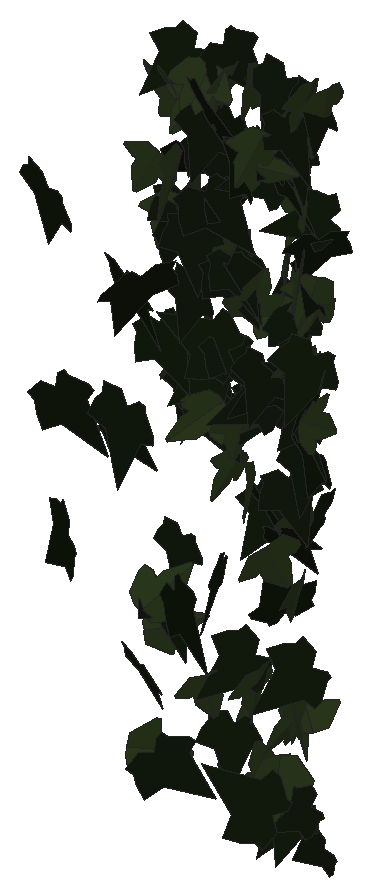
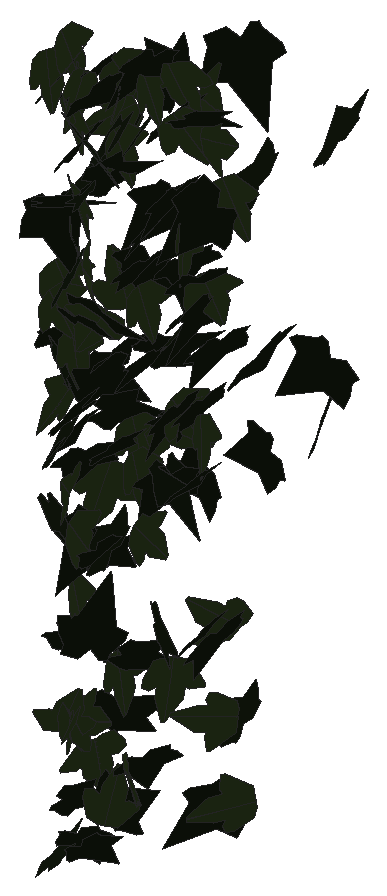
# SketchUp Ruby script. Lengths in inches.
U = 1.inch
M = Sketchup.active_model
def pt(a) = Geom::Point3d.new(a.map { |v| v * U })
def face(e, loops, mat)
  f = e.add_face(loops[0].map { |a| pt(a) })
  loops[1..].each { |l| e.add_face(l.map { |a| pt(a) }).erase! }
  f.material = f.back_material = mat if mat
  f
end
# faces: each face lists its corners as indices into pts; further lists are holes
def faces(e, pts, list, mat = nil) = list.each { |f| face(e, (f[0].is_a?(Array) ? f : [f]).map { |l| l.map { |i| pts[i] } }, mat) }
# xy, xz, yz: faces in a plane at the given z, y or x. An outline is a flat list of corners, or four numbers for a rectangle; further outlines are holes
def ring(l) = l.size == 4 ? [[l[0], l[1]], [l[2], l[1]], [l[2], l[3]], [l[0], l[3]]] : l.each_slice(2).to_a
def flat(e, list, mat, &to3) = list.each { |f| face(e, (f[0].is_a?(Array) ? f : [f]).map { |l| ring(l).map { |u, v| to3.(u, v) } }, mat) }
def xy(e, z, list, mat = nil) = flat(e, list, mat) { |x, y| [x, y, z] }
def xz(e, y, list, mat = nil) = flat(e, list, mat) { |x, z| [x, y, z] }
def yz(e, x, list, mat = nil) = flat(e, list, mat) { |y, z| [x, y, z] }
def lines(e, pts, list) = list.each { |a, b| e.add_line(pt(pts[a]), pt(pts[b])) }
# prism: a flat outline (further loops are holes) pulled along v
def prism(e, loops, v, mat = nil)
  f = face(e, loops, mat); d = Geom::Vector3d.new(v.map { |x| x * U })
  f.pushpull(f.normal.samedirection?(d) ? d.length : -d.length)
end
def box(e, o, s, mat = nil) = prism(e, [[o, [o[0] + s[0], o[1], o[2]], [o[0] + s[0], o[1] + s[1], o[2]], [o[0], o[1] + s[1], o[2]]]], [0, 0, s[2]], mat)
def at(x, y, z, deg = 0) = Geom::Transformation.translation(pt([x, y, z])) * Geom::Transformation.rotation(ORIGIN, Z_AXIS, deg.degrees)
def axes(o, x, y, z) = Geom::Transformation.new([*x, 0, *y, 0, *z, 0, *pt(o).to_a, 1])
def part(name) = M.definitions.add(name)
# library, detail: a bought-in or finely detailed component or shape, given as its bounding box
def library(name, o, s) = part(name).tap { |d| box(d.entities, o, s) }
def detail(e, o, s) = box(e.add_group.entities, o, s)
def put(e, d, t, mat = nil) = e.add_instance(d, t).tap { |i| i.material = mat if mat }
def group(e, t, mat = nil) = e.add_group.tap { |g| g.transformation = t; g.material = mat if mat }.entities
root = M.entities
M.materials.add("efeu1").color = [18, 25, 13]
M.materials.add("efeu2").color = [43, 57, 29]
c1 = part("ivyleaf_9")
p = [[1.54,2.16,1.25],[1.36,2.04,1.19],[-0.21,0.99,0.68],[-0.71,1.11,0.82],[-0.85,0.86,0.67],[-0.8,0.17,0.21],
  [-0.9,-0.01,0.1],[-0.67,-0.16,-0.02],[-0.08,-0.08,-0.05],[-0.03,-0.6,-0.4],[0.65,-0.88,-0.66],[0.83,-0.6,-0.49],
  [1.29,-0.42,-0.43],[1.8125,-0.07,-0.26],[1.21,0.44,0.15]]
faces(c1.entities,p,[[0,1,2,3,4,5,6,7,8,9,10,11,12,13,14]],"efeu1")
c2 = part("ivyleaf_10")
p = [[0,0.5,-0.03],[-0.0625,2.02,-0.43],[-0.19,2.01,-0.46],[-0.54,1.05,-0.29],[-0.52,0.625,-0.18],[-0.83,0.76,-0.28],
  [-1.16,0.64,-0.33],[-1.15,0.33,-0.24],[-0.77,-0.39,0.02],[-0.3,-0.51,0.16],[0.04,-0.48,0.23],[-0.02,2.01,-0.4375],
  [-0.06,2.01,-0.43],[0.04,-0.49,0.23],[0.67,-0.49,0.14],[1.38,0.36,-0.2],[1.375,0.51,-0.24],[0.81,0.65,-0.19],
  [0.62,0.59,-0.15],[0.6,1.09,-0.28],[0.5,1.23,-0.31]]
faces(c2.entities,p,[[0,1,2,3,4,5,6,7,8,9,10],[11,12,0,13,14,15,16,17,18,19,20]],"efeu2")
put(root,c1,axes([535.38,119.04,238.33],[-0.0046,1.10977,-0.65289],[0.01656,-0.65279,-1.10972],[-1.28748,-0.01237,-0.01194]))
put(root,c1,axes([529.95,120.92,223.31],[0.0057,-0.47191,1.12844],[-0.04306,-1.12783,-0.47144],[1.22238,-0.03753,-0.02186]))
put(root,c1,axes([527.55,122.67,238.21],[0.11149,-0.92715,0.85418],[0.28235,-0.81737,-0.92404],[1.22862,0.27197,0.13484]))
put(root,c1,axes([534.18,122.9,221.11],[-0.18366,-0.06917,-1.25975],[1.24507,0.19576,-0.19227],[0.20386,-1.25793,0.03935]))
put(root,c1,axes([531.27,123.22,235.0625],[0.67156,-0.97073,0.50529],[0.29781,-0.40836,-1.18033],[1.05306,0.73454,0.01157]))
put(root,c1,axes([527.59,123.24,228.4375],[-0.22473,-0.1748,-1.15039],[0.8751,0.74683,-0.28443],[0.76691,-0.90341,-0.01255]))
put(root,c1,axes([530.36,124.36,227.99],[0.02553,-1.21276,0.34059],[-0.00472,-0.34075,-1.21297],[1.25966,0.0233,-0.01145]))
put(root,c2,axes([531.97,125.53,239.72],[0.32011,-0.69999,0.92386],[0.52264,-0.76831,-0.76323],[1.03458,0.60472,0.09971]))
put(root,c1,axes([536.72,125.87,210.3],[-0.83288,-0.68543,-0.49251],[-0.36063,-0.33659,1.07829],[-0.7631,0.90717,0.02796]))
put(root,c2,axes([534.82,127.01,224.86],[0.15571,-0.17233,1.06385],[0.75009,-0.75449,-0.232],[0.77385,0.766,0.01082]))
put(root,c1,axes([527.87,126.68,225.62],[0.10645,-0.11566,-1.01801],[0.9531,0.38672,0.05572],[0.37593,-0.9477,0.14698]))
put(root,c2,axes([534.97,127.39,240.99],[-0.33884,-0.75966,0.57853],[0.0263,-0.62106,-0.80011],[0.9545,-0.25256,0.22742]))
put(root,c1,axes([533.66,127.9,239.13],[0.01708,-0.53645,0.8538],[0.07926,-0.85056,-0.536],[1.00522,0.07618,0.02776]))
put(root,c1,axes([531.83,127.72,241.38],[0.29946,-0.45974,1.03584],[0.57254,-0.86323,-0.54865],[0.97802,0.64611,0.00403]))
put(root,c1,axes([528.4,127.72,213.63],[0.33338,-0.69395,0.64405],[0.39585,-0.51809,-0.76314],[0.86004,0.50746,0.1016]))
put(root,c2,axes([535.88,126.97,221.9],[-0.52924,-0.92173,-0.5177],[0.23506,0.46185,-1.0626],[1.0307,-0.57862,-0.02349]))
put(root,c2,axes([532.3,127.31,214.41],[-0.62681,-0.78763,-0.18353],[0.10161,0.15366,-1.00648],[0.80232,-0.63479,-0.01591]))
put(root,c1,axes([529.69,127.5,230.36],[0.19092,-0.92853,-0.51828],[-0.01311,0.52447,-0.94445],[1.06331,0.17319,0.08142]))
put(root,c2,axes([529.54,127.01,217.43],[0.59273,0.36852,-0.87776],[0.66449,0.58028,0.69234],[0.68171,-0.88604,0.08835]))
put(root,c1,axes([531.49,128.46,240.24],[-0.1705,-0.95111,0.35698],[-0.013,-0.3599,-0.9651],[1.01581,-0.16424,0.04756]))
put(root,c1,axes([530.49,128.65,231.96],[-0.08839,-0.88095,0.40202],[0.03436,-0.40629,-0.88275],[0.96773,-0.06603,0.06806]))
put(root,c2,axes([528.9,128.12,237.77],[-0.85627,-0.23854,0.55865],[-0.50677,-0.25182,-0.88428],[0.33492,-0.9909,0.09024]))
put(root,c1,axes([529.29,128.2,217.5],[0.29353,-1.03921,-0.33354],[-0.09426,0.31996,-1.07986],[1.08735,0.30827,-0.00357]))
put(root,c1,axes([529.375,127.65,209.72],[0.05499,-0.3085,-1.06393],[0.16403,1.05576,-0.29766],[1.09554,-0.14259,0.09798]))
put(root,c1,axes([533.46,128.83,215.38],[-0.74213,-0.57989,0.41159],[-0.31108,-0.27023,-0.94162],[0.63947,-0.80445,0.01961]))
put(root,c2,axes([531.44,128.6875,226.47],[0.49114,0.3893,-0.89438],[-0.69244,-0.56614,-0.62666],[-0.68702,0.8489,-0.00777]))
put(root,c2,axes([528.55,127.5625,209.76],[0.06404,0.17176,1.08411],[0.49196,0.96628,-0.18216],[-0.98121,0.49569,-0.02057]))
put(root,c1,axes([532.14,128.66,229.58],[-0.60897,-0.77169,-0.49184],[-0.29953,-0.39015,0.98301],[-0.86469,0.67862,0.00586]))
put(root,c2,axes([531.23,128.42,242.49],[1.05194,0.26422,-0.32485],[-0.31331,-0.0861,-1.08459],[-0.27781,1.09758,-0.00688]))
put(root,c2,axes([534.27,127.84,239.5],[-0.28997,-0.29863,-0.92444],[0.72371,0.57719,-0.41346],[0.64809,-0.77815,0.04809]))
put(root,c2,axes([533.94,128.53,214.65],[-0.07636,-1.02546,-0.052],[0.0077,0.05157,-1.02829],[1.02675,-0.07665,0.00384]))
put(root,c1,axes([536.29,129.125,215.61],[-0.83413,-0.54906,0.36469],[-0.30431,-0.20099,-0.99862],[0.58469,-0.88791,0.00053]))
put(root,c1,axes([533.87,129.19,229],[-0.16961,-0.91761,0.26402],[-0.02435,-0.26391,-0.93287],[0.95453,-0.16979,0.02312]))
put(root,c2,axes([535.03,128.69,210.55],[0.49474,1.02493,-0.23982],[-0.13686,-0.20011,-1.13753],[-1.04368,0.51209,0.03548]))
put(root,c1,axes([532.42,128.59,233.62],[-0.31921,-0.43545,-0.83254],[0.4673,0.68923,-0.53967],[0.81509,-0.56568,-0.01665]))
put(root,c1,axes([530.22,129.03,234.58],[-0.1481,-0.94071,-0.24912],[0.05965,0.24274,-0.95208],[0.97131,-0.15834,0.02049]))
put(root,c1,axes([534.11,128.74,208.03],[0.07404,-0.06142,0.97578],[-0.83918,0.49814,0.09503],[-0.50169,-0.8423,-0.01495]))
put(root,c1,axes([531.33,128.51,236.76],[-0.16708,-0.45154,-1.02055],[0.37043,0.95098,-0.4814],[1.05271,-0.4063,0.00742]))
put(root,c2,axes([530.42,129.16,240.74],[-0.66955,-0.43263,0.6152],[-0.38594,-0.5093,-0.7782],[0.64551,-0.75324,0.17283]))
put(root,c1,axes([535.125,128.97,241.36],[0.31032,-0.92507,-0.29054],[-0.00669,0.30301,-0.97191],[0.9696,0.29816,0.08628]))
put(root,c1,axes([532.08,129.39,240.08],[0.29615,-0.93341,0.30808],[0.05897,-0.30431,-0.97867],[0.98117,0.30002,-0.03417]))
put(root,c2,axes([533.38,128.95,231.9],[-0.55454,-0.86595,0.15564],[0.09428,0.12443,1.02822],[-0.87476,0.56237,0.01215]))
put(root,c1,axes([532.13,129.29,211.35],[-0.28017,-0.89858,-0.19709],[0.08838,0.17879,-0.94075],[0.91569,-0.29219,0.0305]))
put(root,c1,axes([532.29,129.04,233.75],[0.24414,-0.9025,-0.38384],[0.05874,0.4083,-0.92265],[0.97898,0.20057,0.15108]))
put(root,c1,axes([530.76,129.72,227.65],[-0.58344,-0.56341,0.51119],[-0.15324,-0.54397,-0.77445],[0.74516,-0.553,0.24099]))
put(root,c1,axes([531.9,128.87,229.6875],[0.38285,-0.74033,-0.48948],[0.00691,0.53555,-0.80461],[0.88749,0.3152,0.21741]))
put(root,c2,axes([533.38,129.27,238.99],[-0.0339,-0.98735,0.19467],[0.00157,-0.19483,-0.9879],[1.00636,-0.03296,0.0081]))
put(root,c1,axes([535.17,129.18,224.15],[-0.0756,-0.83801,-0.48407],[0.11167,0.47475,-0.83931],[0.96131,-0.12105,0.05943]))
put(root,c2,axes([532.61,129.25,226.15],[-0.37545,-0.88251,0.1429],[-0.02207,-0.1458,-0.95836],[0.89373,-0.37433,0.03637]))
put(root,c2,axes([531.86,129.39,242.28],[0.12631,-0.97591,0.1992],[0.05774,-0.19328,-0.98354],[0.99436,0.13519,0.03181]))
put(root,c1,axes([533.51,129.9375,238.88],[-0.13909,-0.58411,0.79595],[0.1714,-0.80589,-0.56145],[0.97229,0.05851,0.21284]))
put(root,c1,axes([535.66,129.86,208.48],[-0.52366,-0.43526,0.55721],[-0.41278,-0.37476,-0.68067],[0.57405,-0.66652,0.01885]))
put(root,c2,axes([529.05,128.9,240.47],[-0.21486,0.20824,-1.01826],[-0.85423,0.55692,0.29414],[0.59204,0.87912,0.05486]))
put(root,c2,axes([534.8125,129.99,212.38],[0.08982,-0.36941,0.91137],[0.1727,-0.89501,-0.3798],[0.96811,0.19394,-0.0168]))
put(root,c1,axes([535.5,129.85,225.12],[0.03294,-0.92582,0.25483],[0.00035,-0.25496,-0.92636],[0.96024,0.03185,-0.00841]))
put(root,c2,axes([535.79,129.57,242.77],[0.11025,-0.99371,0.21264],[0.00582,-0.21327,-0.99966],[1.01619,0.10903,-0.01734]))
put(root,c1,axes([534.34,129.82,228.51],[0.01927,0.08127,-0.98957],[-0.16612,-0.97554,-0.08335],[-0.97891,0.16715,-0.00533]))
put(root,c1,axes([535.83,129.9,229.92],[-0.52048,-0.91662,0.05668],[-0.02161,-0.05291,-1.05405],[0.91811,-0.52087,0.00732]))
put(root,c2,axes([529.84,129.94,228.39],[-0.18644,-0.82675,0.56035],[0.08702,-0.5813,-0.82872],[0.99495,-0.10408,0.17748]))
put(root,c1,axes([533.43,130.11,227.1],[-0.64019,-0.42327,0.61702],[-0.52344,-0.32692,-0.76736],[0.53468,-0.82684,-0.01245]))
put(root,c2,axes([535.18,129.89,234.24],[0.63506,-0.61955,0.52491],[0.39646,-0.34497,-0.88683],[0.70865,0.74821,0.02576]))
put(root,c1,axes([531.25,129.55,236.34],[0.46927,-0.83407,-0.32072],[-0.08109,0.32102,-0.95348],[0.88993,0.46907,0.08224]))
put(root,c1,axes([530.9,129.98,218.2],[-0.58223,0.1107,-0.80949],[0.74627,-0.33256,-0.58224],[-0.33257,-0.94004,0.11065]))
put(root,c1,axes([528.82,129.74,228.92],[0.28021,-0.88036,-0.34094],[-0.05675,0.33929,-0.92274],[0.94237,0.28221,0.04581]))
put(root,c1,axes([528.99,130.4,242.05],[-0.78669,-0.55301,0.30356],[-0.09948,-0.37041,-0.93261],[0.62295,-0.75752,0.23441]))
put(root,c2,axes([532.95,129.3,242.21],[0.28662,-0.72547,-0.63623],[0.09197,0.68123,-0.73534],[0.96054,0.15126,0.26026]))
put(root,c1,axes([528.55,130.3,218.625],[0.00391,-0.86888,0.3021],[0.0609,-0.30119,-0.86707],[0.91788,0.02369,0.05624]))
put(root,c1,axes([528.75,129.03,237.47],[0.81404,0.6646,0.32649],[0.23738,0.22536,-1.05062],[-0.70138,0.84762,0.02334]))
put(root,c2,axes([528.35,130.09,234.56],[-0.60935,-0.6876,0.3941],[-0.04175,-0.46858,-0.8821],[0.79144,-0.55413,0.2569]))
put(root,c1,axes([533.64,130.52,237.67],[-0.50991,-0.35208,0.84626],[-0.5977,-0.60644,-0.61245],[0.69488,-0.77999,0.09419]))
put(root,c1,axes([531.58,129.45,243.46],[0.29141,-0.61004,-0.77942],[-0.09534,0.79142,-0.65508],[0.98517,0.25704,0.16715]))
put(root,c1,axes([535.43,130.57,224.93],[0.05667,-0.73281,0.71531],[0.12795,-0.70573,-0.73313],[1.01603,0.12975,0.05243]))
put(root,c2,axes([528.04,129.29,214.66],[0.07876,0.0606,-1.05258],[0.85603,0.6125,0.09932],[0.61548,-0.85964,-0.00344]))
put(root,c2,axes([535.13,129.98,229.58],[-0.17513,-0.95781,0.01471],[-0.00237,-0.01452,-0.97369],[0.95792,-0.17515,0.00028]))
put(root,c2,axes([533.16,130.35,208.99],[-0.52553,-0.72732,-0.37064],[-0.22149,-0.29722,0.8973],[-0.78569,0.57028,-0.00504]))
put(root,c1,axes([535.41,130.66,241.75],[0.09253,-0.90579,0.4396],[0.11104,-0.42958,-0.90851],[1.00068,0.13142,0.06016]))
put(root,c1,axes([535.84,130.27,229.02],[-0.7807,0.30952,-0.54833],[0.51516,-0.18822,-0.83973],[-0.36205,-0.93527,-0.01247]))
put(root,c2,axes([528.66,129.9,227.87],[0.15308,-0.90323,-0.35006],[-0.03501,0.34901,-0.91584],[0.96806,0.15545,0.02224]))
put(root,c1,axes([529.96,130,238.18],[0.3506,-0.76629,-0.51433],[-0.1109,0.51122,-0.83726],[0.91621,0.35511,0.09547]))
put(root,c2,axes([534.98,130.02,212.65],[-0.40367,0.89574,-0.10741],[0.04314,-0.09837,-0.98249],[-0.90112,-0.40596,0.00108]))
put(root,c2,axes([529.5625,129.85,236.32],[0.11842,-0.85591,-0.4873],[-0.056,0.48417,-0.86401],[0.98331,0.13065,0.00948]))
put(root,c1,axes([535.59,130.88,206.04],[-0.43929,-0.37476,0.71593],[0.04718,-0.82538,-0.4031],[0.8067,-0.1558,0.41343]))
put(root,c2,axes([534.86,129.82,241.39],[-0.07803,-0.85517,-0.54167],[0.1664,0.52505,-0.85291],[0.99852,-0.15433,0.09981]))
put(root,c2,axes([535,130.46,212.99],[0.07565,-0.88661,0.28067],[0.06437,-0.27593,-0.88899],[0.92775,0.09144,0.03879]))
put(root,c1,axes([534.42,130.5625,207.64],[-0.57701,-0.63215,-0.13567],[0.10695,0.08602,-0.85565],[0.63764,-0.58647,0.02074]))
put(root,c2,axes([535.07,130.3,240.31],[0.89653,-0.46798,-0.03156],[-0.02645,0.01753,-1.01132],[0.4683,0.89692,0.00329]))
put(root,c1,axes([534.35,129.75,221.08],[0.91739,0.37331,-0.16882],[-0.16026,-0.05405,-0.99038],[-0.37707,0.93122,0.0102]))
put(root,c1,axes([528.48,130.36,234.92],[-0.18038,-0.85108,-0.41918],[0.11055,0.40493,-0.86971],[0.94224,-0.21044,0.02179]))
put(root,c1,axes([534.42,130.21,231.27],[-0.67562,0.28963,0.67405],[-0.65705,0.16875,-0.73109],[-0.32636,-0.93933,0.07649]))
put(root,c2,axes([535.43,130.52,232.92],[-0.48129,-0.73926,0.36851],[-0.05202,-0.39853,-0.86741],[0.82438,-0.45674,0.16041]))
put(root,c2,axes([534.74,130.33,236.66],[0.84057,-0.56842,-0.03707],[-0.02994,0.02189,-1.01471],[0.56884,0.8411,0.00136]))
put(root,c1,axes([536,130.11,235.48],[0.1786,0.81012,-0.57667],[-0.13455,-0.56082,-0.82953],[-0.98526,0.22344,0.00875]))
put(root,c2,axes([534.375,130.7,221.44],[0.18269,-0.89521,0.50998],[0.07367,-0.50526,-0.91332],[1.02765,0.19537,-0.02519]))
put(root,c1,axes([534.75,131.01,226.64],[-0.28059,-0.72294,0.61402],[-0.08647,-0.61816,-0.76733],[0.94455,-0.27135,0.11215]))
put(root,c1,axes([533.51,130.97,241.84],[-0.25326,-1.00816,0.31724],[-0.04912,-0.31464,-1.03912],[1.05576,-0.25648,0.02776]))
put(root,c2,axes([534.7,130.34,218.48],[0.21633,-0.90661,-0.06868],[-0.01932,0.06599,-0.93206],[0.90901,0.21716,-0.00347]))
put(root,c1,axes([533.79,130.42,237.67],[0.67664,-0.73378,0.06745],[0.06241,-0.03417,-0.99788],[0.73423,0.67913,0.02267]))
put(root,c1,axes([533.94,130.82,207.39],[-0.53882,-0.65567,0.16211],[-0.10339,-0.12486,-0.84866],[0.66745,-0.54865,-0.00059]))
put(root,c2,axes([535.57,129.67,222.46],[-0.13336,0.62433,-0.79285],[-0.14085,0.7804,0.63822],[0.99928,0.19332,-0.01585]))
put(root,c1,axes([534.45,130.75,231.25],[-0.70271,-0.47324,-0.42634],[0.48167,0.02059,-0.81676],[0.41679,-0.82167,0.22509]))
put(root,c2,axes([533.6,130.14,231.28],[0.71665,0.48313,0.53213],[0.42882,0.31563,-0.86409],[-0.57679,0.83494,0.01874]))
put(root,c1,axes([535.83,130.89,236.07],[-0.79394,-0.03572,0.5529],[-0.47871,-0.44221,-0.71596],[0.27896,-0.86052,0.34498]))
put(root,c2,axes([531.78,130.69,211.35],[0.68998,-0.55647,0.39251],[0.29251,-0.2624,-0.88621],[0.61494,0.74918,-0.01885]))
put(root,c1,axes([534.2,130.79,239.27],[0.22462,-0.96117,0.10089],[0.02364,-0.09808,-0.98707],[0.96616,0.22586,0.0007]))
put(root,c1,axes([534.83,131.07,232.6],[0.02329,-0.61386,0.74538],[0.16489,-0.73212,-0.60809],[0.95144,0.14191,0.08713]))
put(root,c2,axes([535.86,129.65,226.88],[-0.02693,0.50115,0.88677],[-0.22538,0.86216,-0.49409],[-0.99334,-0.20921,0.08806]))
put(root,c2,axes([531.51,130.54,225.45],[0.03829,-1.01028,0.05909],[0.00716,-0.05886,-1.011],[1.01199,0.03864,0.00491]))
put(root,c1,axes([528.33,130.03,233.71],[0.38254,-0.53879,-0.81678],[-0.35139,0.74284,-0.65459],[0.91321,0.51153,0.09027]))
put(root,c2,axes([536.03,130.49,242.18],[-0.17848,-0.99942,-0.03547],[0.01155,0.03397,-1.01521],[0.99998,-0.17878,0.0054]))
put(root,c1,axes([532.49,130.96,221.48],[0.36952,-0.7475,0.65713],[0.37994,-0.54193,-0.83011],[0.9199,0.5241,0.07889]))
put(root,c2,axes([535.3,130.41,212.26],[0.73767,0.6168,0.26162],[-0.21433,-0.15143,0.96134],[0.63479,-0.7679,0.02056]))
put(root,c1,axes([529.55,130.43,228.65],[0.37676,-0.84763,-0.49417],[-0.1854,0.45831,-0.92748],[0.96349,0.41965,0.01477]))
put(root,c2,axes([530.83,131.02,222.81],[-0.03172,-0.71298,0.61435],[0.04899,-0.61512,-0.71134],[0.93988,0.008,0.05782]))
put(root,c1,axes([533.57,130.85,216.6875],[0.58353,0.35379,0.7817],[-0.66758,-0.40669,0.68241],[0.53904,-0.88666,-0.00109]))
put(root,c1,axes([529.92,130.52,225.75],[-0.56238,0.81357,-0.37128],[0.21559,-0.30232,-0.98901],[-0.86791,-0.60227,-0.00509]))
put(root,c1,axes([528.76,130.7,233.08],[0.47501,-0.83569,-0.09748],[-0.01808,0.10178,-0.96064],[0.84116,0.47411,0.03439]))
put(root,c2,axes([533.62,131.05,233.79],[0.39793,-0.4455,0.75595],[0.55689,-0.51324,-0.59561],[0.6781,0.68294,0.04552]))
put(root,c1,axes([528.43,131.19,225.87],[-0.15538,-0.87167,0.31214],[0.07954,-0.3279,-0.8761],[0.92245,-0.11856,0.12812]))
put(root,c2,axes([535.29,130.98,231.81],[-0.24703,-0.83242,0.43741],[0.05237,-0.46372,-0.85293],[0.93889,-0.19315,0.16266]))
put(root,c1,axes([529.88,130.43,225.48],[-0.01868,-0.69935,-0.72406],[0.05163,0.72256,-0.69924],[1.00533,-0.0501,0.02246]))
put(root,c1,axes([534.62,130.34,239.45],[-0.67322,0.63694,0.39748],[-0.30425,0.25662,-0.92654],[-0.68637,-0.73848,0.02084]))
put(root,c1,axes([532.32,131.29,226.21],[-0.35803,-0.76557,0.37904],[-0.01946,-0.40356,-0.83349],[0.85404,-0.33014,0.13991]))
put(root,c1,axes([532.9,131.21,221.41],[-0.53412,-0.7798,0.21363],[-0.12673,-0.17213,-0.94516],[0.79854,-0.5489,-0.00711]))
put(root,c2,axes([530.96,130.84,233.39],[-0.14699,-0.94789,0.18202],[-0.00038,-0.18406,-0.95883],[0.9652,-0.14442,0.02734]))
put(root,c1,axes([535.8,130.58,222.12],[-0.73239,0.67531,-0.07106],[0.05041,-0.05015,-0.99621],[-0.67716,-0.73412,0.00269]))
